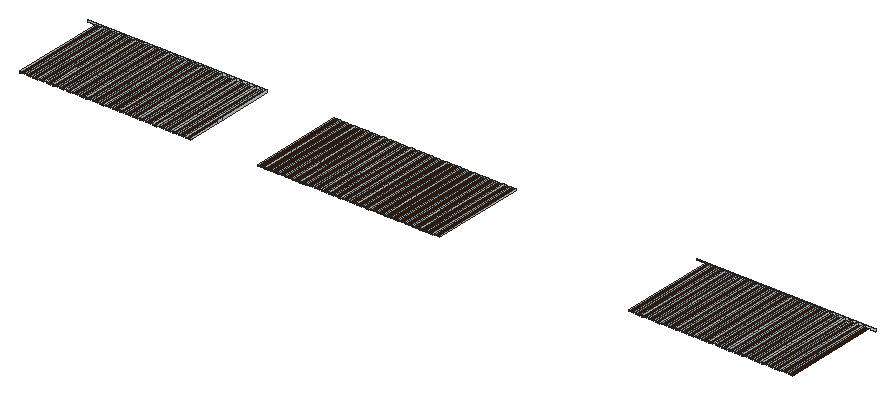
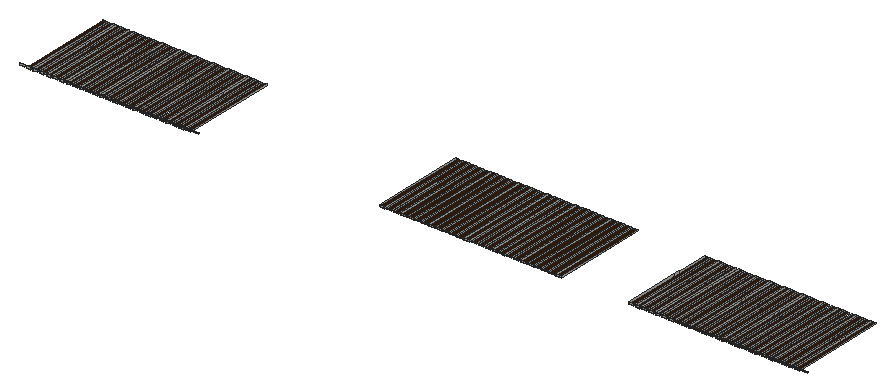
# SketchUp Ruby script. Lengths in inches.
U = 1.inch
M = Sketchup.active_model
def pt(a) = Geom::Point3d.new(a.map { |v| v * U })
def face(e, loops, mat)
  f = e.add_face(loops[0].map { |a| pt(a) })
  loops[1..].each { |l| e.add_face(l.map { |a| pt(a) }).erase! }
  f.material = f.back_material = mat if mat
  f
end
# faces: each face lists its corners as indices into pts; further lists are holes
def faces(e, pts, list, mat = nil) = list.each { |f| face(e, (f[0].is_a?(Array) ? f : [f]).map { |l| l.map { |i| pts[i] } }, mat) }
# xy, xz, yz: faces in a plane at the given z, y or x. An outline is a flat list of corners, or four numbers for a rectangle; further outlines are holes
def ring(l) = l.size == 4 ? [[l[0], l[1]], [l[2], l[1]], [l[2], l[3]], [l[0], l[3]]] : l.each_slice(2).to_a
def flat(e, list, mat, &to3) = list.each { |f| face(e, (f[0].is_a?(Array) ? f : [f]).map { |l| ring(l).map { |u, v| to3.(u, v) } }, mat) }
def xy(e, z, list, mat = nil) = flat(e, list, mat) { |x, y| [x, y, z] }
def xz(e, y, list, mat = nil) = flat(e, list, mat) { |x, z| [x, y, z] }
def yz(e, x, list, mat = nil) = flat(e, list, mat) { |y, z| [x, y, z] }
def lines(e, pts, list) = list.each { |a, b| e.add_line(pt(pts[a]), pt(pts[b])) }
# prism: a flat outline (further loops are holes) pulled along v
def prism(e, loops, v, mat = nil)
  f = face(e, loops, mat); d = Geom::Vector3d.new(v.map { |x| x * U })
  f.pushpull(f.normal.samedirection?(d) ? d.length : -d.length)
end
def box(e, o, s, mat = nil) = prism(e, [[o, [o[0] + s[0], o[1], o[2]], [o[0] + s[0], o[1] + s[1], o[2]], [o[0], o[1] + s[1], o[2]]]], [0, 0, s[2]], mat)
def at(x, y, z, deg = 0) = Geom::Transformation.translation(pt([x, y, z])) * Geom::Transformation.rotation(ORIGIN, Z_AXIS, deg.degrees)
def axes(o, x, y, z) = Geom::Transformation.new([*x, 0, *y, 0, *z, 0, *pt(o).to_a, 1])
def part(name) = M.definitions.add(name)
# library, detail: a bought-in or finely detailed component or shape, given as its bounding box
def library(name, o, s) = part(name).tap { |d| box(d.entities, o, s) }
def detail(e, o, s) = box(e.add_group.entities, o, s)
def put(e, d, t, mat = nil) = e.add_instance(d, t).tap { |i| i.material = mat if mat }
def group(e, t, mat = nil) = e.add_group.tap { |g| g.transformation = t; g.material = mat if mat }.entities
root = M.entities
M.materials.add("[Wood Veneer 01]").color = [51, 28, 15]
xy(root,503.875,[[253.94,246.64,259.43,361.27],[261.94,246.64,267.43,361.27],[269.94,246.64,275.43,361.27],[277.94,246.64,283.43,361.27],[285.94,246.64,291.43,361.27],
  [293.94,246.64,299.43,361.27],[301.94,246.64,307.43,361.27],[309.94,246.64,315.43,361.27],[987.51,246.64,993,361.27],[995.51,246.64,1001,361.27],
  [1003.51,246.64,1009,361.27],[1011.51,246.64,1017,361.27],[1019.51,246.64,1025,361.27],[1027.51,246.64,1033,361.27],[1035.51,246.64,1041,361.27]],"[Wood Veneer 01]")
xy(root,504,[[171.43,283.7,171.43,288.72,172.08,288.63,172.69,288.38,173.21,287.98,173.61,287.46,173.86,286.86,173.94,286.21,173.86,285.56,173.61,284.95,173.21,284.43,172.69,284.03,172.08,283.78],[905,283.7,905,288.72,905.65,288.63,906.25,288.38,906.77,287.98,907.17,287.46,907.42,286.86,907.51,286.21,907.42,285.56,907.17,284.95,906.77,284.43,906.25,284.03,905.65,283.78]])
xy(root,504,[[109.94,246.64,115.43,361.27],[117.94,246.64,123.43,361.27],[125.94,246.64,131.43,361.27],[133.94,246.64,139.43,361.27],[141.94,246.64,147.43,361.27],
  [149.94,246.64,155.43,361.27],[157.94,246.64,163.43,361.27],[165.94,246.64,165.94,361.27,171.43,361.27,171.43,288.72,170.79,288.63,170.18,288.38,169.66,287.98,169.26,287.46,169.01,286.86,168.92,286.21,169.01,285.56,169.26,284.95,169.66,284.43,170.18,284.03,170.79,283.78,171.43,283.7,171.43,246.64],[173.94,246.64,179.43,361.27],[181.94,246.64,187.43,361.27],
  [189.94,246.64,195.43,361.27],[197.94,246.64,203.43,361.27],[205.94,246.64,211.43,361.27],[213.94,246.64,219.43,361.27],[221.94,246.64,227.43,361.27],
  [229.94,246.64,235.43,361.27],[237.94,246.64,243.43,361.27],[245.94,246.64,251.43,361.27],[396.57,246.64,403.28,361.27],[405.07,246.64,411.78,361.27],
  [413.57,246.64,420.28,361.27],[422.07,246.64,428.78,361.27],[430.57,246.64,437.28,361.27],[439.07,246.64,445.78,361.27],[447.57,246.64,454.28,361.27],
  [456.07,246.64,462.78,361.27],[464.57,246.64,471.28,361.27],[473.07,246.64,479.78,361.27],[481.57,246.64,488.28,361.27],[490.07,246.64,496.78,361.27],
  [498.57,246.64,505.28,361.27],[507.07,246.64,513.78,361.27],[515.57,246.64,522.28,361.27],[524.07,246.64,530.78,361.27],[532.57,246.64,539.28,361.27],
  [541.07,246.64,547.78,361.27],[549.57,246.64,556.28,361.27],[558.07,246.64,564.78,361.27],[566.57,246.64,573.28,361.27],[575.07,246.64,581.78,361.27],
  [583.57,246.64,590.28,361.27],[592.07,246.64,598.78,361.27],[600.57,246.64,607.28,361.27],[609.07,246.64,615.78,361.27],[843.51,246.64,849,361.27],
  [851.51,246.64,857,361.27],[859.51,246.64,865,361.27],[867.51,246.64,873,361.27],[875.51,246.64,881,361.27],[883.51,246.64,889,361.27],
  [891.51,246.64,897,361.27],[899.51,246.64,899.51,361.27,905,361.27,905,288.72,904.35,288.63,903.74,288.38,903.22,287.98,902.82,287.46,902.57,286.86,902.49,286.21,902.57,285.56,902.82,284.95,903.22,284.43,903.74,284.03,904.35,283.78,905,283.7,905,246.64],[907.51,246.64,913,361.27],[915.51,246.64,921,361.27],[923.51,246.64,929,361.27],
  [931.51,246.64,937,361.27],[939.51,246.64,945,361.27],[947.51,246.64,953,361.27],[955.51,246.64,961,361.27],[963.51,246.64,969,361.27],
  [971.51,246.64,977,361.27],[979.51,246.64,985,361.27],[171.43,283.7,170.79,283.78,170.18,284.03,169.66,284.43,169.26,284.95,169.01,285.56,168.92,286.21,169.01,286.86,169.26,287.46,169.66,287.98,170.18,288.38,170.79,288.63,171.43,288.72],[905,283.7,904.35,283.78,903.74,284.03,903.22,284.43,902.82,284.95,902.57,285.56,902.49,286.21,902.57,286.86,902.82,287.46,903.22,287.98,903.74,288.38,904.35,288.63,905,288.72]],"[Wood Veneer 01]")
xz(root,246.64,[[253.94,503.875,259.43,505.1875],[261.94,503.875,267.43,503.875,267.43,505.21,261.94,505.19],[269.94,503.875,275.43,503.875,275.43,505.22,269.94,505.21],[277.94,503.875,283.43,503.875,283.43,505.24,277.94,505.23],[285.94,503.875,291.43,503.875,291.43,505.26,285.94,505.25],
  [293.94,503.875,299.43,503.875,299.43,505.28,293.94,505.26],[301.94,503.875,307.43,503.875,307.43,505.29,301.94,505.28],[309.94,503.875,315.43,503.875,315.43,505.3125,309.94,505.3],[987.51,503.875,993,505.1875],[995.51,503.875,1001,503.875,1001,505.21,995.51,505.19],
  [1003.51,503.875,1009,503.875,1009,505.22,1003.51,505.21],[1011.51,503.875,1017,503.875,1017,505.24,1011.51,505.23],[1019.51,503.875,1025,503.875,1025,505.26,1019.51,505.25],[1027.51,503.875,1033,503.875,1033,505.28,1027.51,505.26],[1035.51,503.875,1041,503.875,1041,505.29,1035.51,505.28],
  [109.94,504,115.43,505.3125],[117.94,504,123.43,505.3125],[125.94,504,131.43,505.3125],[133.94,504,139.43,505.3125],[141.94,504,147.43,505.3125],
  [149.94,504,155.43,505.3125],[157.94,504,163.43,505.3125],[165.94,504,171.43,505.3125],[173.94,504,179.43,505.3125],[181.94,504,187.43,505.3125],
  [189.94,504,195.43,505.3125],[197.94,504,203.43,505.3125],[205.94,504,211.43,505.3125],[213.94,504,219.43,505.3125],[221.94,504,227.43,505.3125],
  [229.94,504,235.43,505.3125],[237.94,504,243.43,505.3125],[245.94,504,251.43,505.3125],[396.57,504,403.28,505.3125],[405.07,504,411.78,505.3125],
  [413.57,504,420.28,505.3125],[422.07,504,428.78,505.3125],[430.57,504,437.28,505.3125],[439.07,504,445.78,505.3125],[447.57,504,454.28,505.3125],
  [456.07,504,462.78,505.3125],[464.57,504,471.28,505.3125],[473.07,504,479.78,505.3125],[481.57,504,488.28,505.3125],[490.07,504,496.78,505.3125],
  [498.57,504,505.28,505.3125],[507.07,504,513.78,505.3125],[515.57,504,522.28,505.3125],[524.07,504,530.78,505.3125],[532.57,504,539.28,505.3125],
  [541.07,504,547.78,505.3125],[549.57,504,556.28,505.3125],[558.07,504,564.78,505.3125],[566.57,504,573.28,505.3125],[575.07,504,581.78,505.3125],
  [583.57,504,590.28,505.3125],[592.07,504,598.78,505.3125],[600.57,504,607.28,505.3125],[609.07,504,615.78,505.3125],[843.51,504,849,505.3125],
  [851.51,504,857,505.3125],[859.51,504,865,505.3125],[867.51,504,873,505.3125],[875.51,504,881,505.3125],[883.51,504,889,505.3125],
  [891.51,504,897,505.3125],[899.51,504,905,505.3125],[907.51,504,913,505.3125],[915.51,504,921,505.3125],[923.51,504,929,505.3125],
  [931.51,504,937,505.3125],[939.51,504,945,505.3125],[947.51,504,953,505.3125],[955.51,504,961,505.3125],[963.51,504,969,505.3125],
  [971.51,504,977,505.3125],[979.51,504,985,505.3125]],"[Wood Veneer 01]")
xz(root,361.27,[[261.94,503.875,267.43,503.875,267.43,505.3125,269.94,505.3125,269.94,503.875,275.43,503.875,275.43,505.3125,277.94,505.3125,277.94,503.875,283.43,503.875,283.43,505.3125,285.94,505.3125,285.94,503.875,291.43,503.875,291.43,505.3125,293.94,505.3125,293.94,503.875,299.43,503.875,299.43,505.3125,301.94,505.3125,301.94,503.875,307.43,503.875,307.43,505.3125,309.94,505.3125,309.94,503.875,315.43,503.875,315.43,506.8125,100.18,506.8125,100.18,505.3125,253.94,505.3125,253.94,505.1875,259.43,505.1875,259.43,505.3125,261.94,505.3125],[253.94,503.875,259.43,505.1875],[995.51,503.875,1001,503.875,1001,505.3125,1003.51,505.3125,1003.51,503.875,1009,503.875,1009,505.3125,1011.51,505.3125,1011.51,503.875,1017,503.875,1017,505.3125,1019.51,505.3125,1019.51,503.875,1025,503.875,1025,505.3125,1027.51,505.3125,1027.51,503.875,1033,503.875,1033,505.3125,1035.51,505.3125,1035.51,503.875,1041,503.875,1041,505.3125,1043.51,505.3125,1043.51,503.875,1049,503.875,1049,506.8125,833.74,506.8125,833.74,505.3125,987.51,505.3125,987.51,505.1875,993,505.1875,993,505.3125,995.51,505.3125],[987.51,503.875,993,505.1875],[109.94,504,115.43,505.3125],
  [117.94,504,123.43,505.3125],[125.94,504,131.43,505.3125],[133.94,504,139.43,505.3125],[141.94,504,147.43,505.3125],[149.94,504,155.43,505.3125],
  [157.94,504,163.43,505.3125],[165.94,504,171.43,505.3125],[173.94,504,179.43,505.3125],[181.94,504,187.43,505.3125],[189.94,504,195.43,505.3125],
  [197.94,504,203.43,505.3125],[205.94,504,211.43,505.3125],[213.94,504,219.43,505.3125],[221.94,504,227.43,505.3125],[229.94,504,235.43,505.3125],
  [237.94,504,243.43,505.3125],[245.94,504,251.43,505.3125],[396.57,504,403.28,505.3125],[405.07,504,411.78,505.3125],[413.57,504,420.28,505.3125],
  [422.07,504,428.78,505.3125],[430.57,504,437.28,505.3125],[439.07,504,445.78,505.3125],[447.57,504,454.28,505.3125],[456.07,504,462.78,505.3125],
  [464.57,504,471.28,505.3125],[473.07,504,479.78,505.3125],[481.57,504,488.28,505.3125],[490.07,504,496.78,505.3125],[498.57,504,505.28,505.3125],
  [507.07,504,513.78,505.3125],[515.57,504,522.28,505.3125],[524.07,504,530.78,505.3125],[532.57,504,539.28,505.3125],[541.07,504,547.78,505.3125],
  [549.57,504,556.28,505.3125],[558.07,504,564.78,505.3125],[566.57,504,573.28,505.3125],[575.07,504,581.78,505.3125],[583.57,504,590.28,505.3125],
  [592.07,504,598.78,505.3125],[600.57,504,607.28,505.3125],[609.07,504,614.76,505.3125],[614.76,504,615.78,505.3125],[843.51,504,849,505.3125],
  [851.51,504,857,505.3125],[859.51,504,865,505.3125],[867.51,504,873,505.3125],[875.51,504,881,505.3125],[883.51,504,889,505.3125],
  [891.51,504,897,505.3125],[899.51,504,905,505.3125],[907.51,504,913,505.3125],[915.51,504,921,505.3125],[923.51,504,929,505.3125],
  [931.51,504,937,505.3125],[939.51,504,945,505.3125],[947.51,504,953,505.3125],[955.51,504,961,505.3125],[963.51,504,969,505.3125],
  [971.51,504,977,505.3125],[979.51,504,985,505.3125]])
yz(root,109.94,[[246.64,504,361.27,505.3125]])
yz(root,115.43,[[246.64,504,286.21,505.3125],[286.21,504,293.45,505.3125],[293.45,504,293.46,505.3125],[293.46,504,361.27,505.3125]])
yz(root,117.94,[[246.64,504,361.27,505.3125]])
yz(root,123.43,[[246.64,504,286.21,505.3125],[286.21,504,293.45,505.3125],[293.45,504,293.46,505.3125],[293.46,504,361.27,505.3125]])
yz(root,125.94,[[246.64,504,361.27,505.3125]])
yz(root,131.43,[[246.64,504,286.21,505.3125],[286.21,504,293.45,505.3125],[293.45,504,293.46,505.3125],[293.46,504,361.27,505.3125]])
yz(root,133.94,[[246.64,504,361.27,505.3125]])
yz(root,139.43,[[246.64,504,286.21,505.3125],[286.21,504,293.45,505.3125],[293.45,504,293.46,505.3125],[293.46,504,361.27,505.3125]])
yz(root,141.94,[[246.64,504,361.27,505.3125]])
yz(root,147.43,[[246.64,504,286.21,505.3125],[286.21,504,293.45,505.3125],[293.45,504,293.46,505.3125],[293.46,504,361.27,505.3125]])
yz(root,149.94,[[246.64,504,361.27,505.3125]])
yz(root,155.43,[[246.64,504,286.21,505.3125],[286.21,504,293.45,505.3125],[293.45,504,293.46,505.3125],[293.46,504,361.27,505.3125]])
yz(root,157.94,[[246.64,504,361.27,505.3125]])
yz(root,163.43,[[246.64,504,286.21,505.3125],[286.21,504,293.45,505.3125],[293.45,504,293.46,505.3125],[293.46,504,361.27,505.3125]])
yz(root,165.94,[[246.64,504,361.27,505.3125]])
yz(root,171.43,[[246.64,504,286.21,505.3125],[286.21,504,293.45,505.3125],[293.45,504,293.46,505.3125],[293.46,504,361.27,505.3125]])
yz(root,173.94,[[246.64,504,361.27,505.3125]])
yz(root,179.43,[[246.64,504,286.21,505.3125],[286.21,504,293.45,505.3125],[293.45,504,293.46,505.3125],[293.46,504,361.27,505.3125]])
yz(root,181.94,[[246.64,504,361.27,505.3125]])
yz(root,187.43,[[246.64,504,286.21,505.3125],[286.21,504,293.45,505.3125],[293.45,504,293.46,505.3125],[293.46,504,361.27,505.3125]])
yz(root,189.94,[[246.64,504,361.27,505.3125]])
yz(root,195.43,[[246.64,504,286.21,505.3125],[286.21,504,293.45,505.3125],[293.45,504,293.46,505.3125],[293.46,504,361.27,505.3125]])
yz(root,197.94,[[246.64,504,361.27,505.3125]])
yz(root,203.43,[[246.64,504,286.21,505.3125],[286.21,504,293.45,505.3125],[293.45,504,293.46,505.3125],[293.46,504,361.27,505.3125]])
yz(root,205.94,[[246.64,504,361.27,505.3125]])
yz(root,211.43,[[246.64,504,286.21,505.3125],[286.21,504,293.45,505.3125],[293.45,504,293.46,505.3125],[293.46,504,361.27,505.3125]])
yz(root,213.94,[[246.64,504,361.27,505.3125]])
yz(root,219.43,[[246.64,504,286.21,505.3125],[286.21,504,293.45,505.3125],[293.45,504,293.46,505.3125],[293.46,504,361.27,505.3125]])
yz(root,221.94,[[246.64,504,361.27,505.3125]])
yz(root,227.43,[[246.64,504,286.21,505.3125],[286.21,504,293.45,505.3125],[293.45,504,293.46,505.3125],[293.46,504,361.27,505.3125]])
yz(root,229.94,[[246.64,504,361.27,505.3125]])
yz(root,235.43,[[246.64,504,286.21,505.3125],[286.21,504,293.45,505.3125],[293.45,504,293.46,505.3125],[293.46,504,361.27,505.3125]])
yz(root,237.94,[[246.64,504,361.27,505.3125]])
yz(root,243.43,[[246.64,504,286.21,505.3125],[286.21,504,293.45,505.3125],[293.45,504,293.46,505.3125],[293.46,504,361.27,505.3125]])
yz(root,245.94,[[246.64,504,361.27,505.3125]])
yz(root,251.43,[[246.64,504,286.21,505.3125],[286.21,504,293.45,505.3125],[293.45,504,293.46,505.3125],[293.46,504,361.27,505.3125]])
yz(root,253.94,[[246.64,503.875,361.27,505.1875]])
yz(root,259.43,[[246.64,503.875,286.21,505.1875],[286.21,503.875,293.45,505.1875],[293.45,503.875,293.46,505.1875],[293.46,503.875,361.27,505.1875]])
yz(root,261.94,[[246.64,503.875,361.27,505.3125]])
yz(root,267.43,[[246.64,503.875,286.21,505.3125],[286.21,503.875,293.45,505.3125],[293.45,503.875,293.46,505.3125],[293.46,503.875,361.27,505.3125]])
yz(root,269.94,[[246.64,503.875,361.27,505.3125]])
yz(root,275.43,[[246.64,503.875,286.21,505.3125],[286.21,503.875,293.45,505.3125],[293.45,503.875,293.46,505.3125],[293.46,503.875,361.27,505.3125]])
yz(root,277.94,[[246.64,503.875,361.27,505.3125]])
yz(root,283.43,[[246.64,503.875,286.21,505.3125],[286.21,503.875,293.45,505.3125],[293.45,503.875,293.46,505.3125],[293.46,503.875,361.27,505.3125]])
yz(root,285.94,[[246.64,503.875,361.27,505.3125]])
yz(root,291.43,[[246.64,503.875,286.21,505.3125],[286.21,503.875,293.45,505.3125],[293.45,503.875,293.46,505.3125],[293.46,503.875,361.27,505.3125]])
yz(root,293.94,[[246.64,503.875,361.27,505.3125]])
yz(root,299.43,[[246.64,503.875,286.21,505.3125],[286.21,503.875,293.45,505.3125],[293.45,503.875,293.46,505.3125],[293.46,503.875,361.27,505.3125]])
yz(root,301.94,[[246.64,503.875,361.27,505.3125]])
yz(root,307.43,[[246.64,503.875,286.21,505.3125],[286.21,503.875,293.45,505.3125],[293.45,503.875,293.46,505.3125],[293.46,503.875,361.27,505.3125]])
yz(root,309.94,[[246.64,503.875,361.27,505.3125]])
yz(root,315.43,[[246.64,503.875,286.21,505.3125],[286.21,503.875,293.45,506.8125],[293.45,503.875,293.46,506.8125],[293.46,503.875,361.27,506.8125]])
yz(root,396.57,[[246.64,504,286.21,505.3125],[286.21,504,293.45,505.3125],[293.45,504,361.27,505.3125]])
yz(root,403.28,[[246.64,504,361.27,505.3125]])
yz(root,405.07,[[246.64,504,286.21,505.3125],[286.21,504,293.45,505.3125],[293.45,504,361.27,505.3125]])
yz(root,411.78,[[246.64,504,361.27,505.3125]])
yz(root,413.57,[[246.64,504,286.21,505.3125],[286.21,504,293.45,505.3125],[293.45,504,361.27,505.3125]])
yz(root,420.28,[[246.64,504,361.27,505.3125]])
yz(root,422.07,[[246.64,504,286.21,505.3125],[286.21,504,293.45,505.3125],[293.45,504,361.27,505.3125]])
yz(root,428.78,[[246.64,504,361.27,505.3125]])
yz(root,430.57,[[246.64,504,286.21,505.3125],[286.21,504,293.45,505.3125],[293.45,504,361.27,505.3125]])
yz(root,437.28,[[246.64,504,361.27,505.3125]])
yz(root,439.07,[[246.64,504,286.21,505.3125],[286.21,504,293.45,505.3125],[293.45,504,361.27,505.3125]])
yz(root,445.78,[[246.64,504,361.27,505.3125]])
yz(root,447.57,[[246.64,504,286.21,505.3125],[286.21,504,293.45,505.3125],[293.45,504,361.27,505.3125]])
yz(root,454.28,[[246.64,504,361.27,505.3125]])
yz(root,456.07,[[246.64,504,286.21,505.3125],[286.21,504,293.45,505.3125],[293.45,504,361.27,505.3125]])
yz(root,462.78,[[246.64,504,361.27,505.3125]])
yz(root,464.57,[[246.64,504,286.21,505.3125],[286.21,504,293.45,505.3125],[293.45,504,361.27,505.3125]])
yz(root,471.28,[[246.64,504,361.27,505.3125]])
yz(root,473.07,[[246.64,504,286.21,505.3125],[286.21,504,293.45,505.3125],[293.45,504,361.27,505.3125]])
yz(root,479.78,[[246.64,504,361.27,505.3125]])
yz(root,481.57,[[246.64,504,286.21,505.3125],[286.21,504,293.45,505.3125],[293.45,504,361.27,505.3125]])
yz(root,488.28,[[246.64,504,361.27,505.3125]])
yz(root,490.07,[[246.64,504,286.21,505.3125],[286.21,504,293.45,505.3125],[293.45,504,361.27,505.3125]])
yz(root,496.78,[[246.64,504,361.27,505.3125]])
yz(root,498.57,[[246.64,504,286.21,505.3125],[286.21,504,293.45,505.3125],[293.45,504,361.27,505.3125]])
yz(root,505.28,[[246.64,504,361.27,505.3125]])
yz(root,507.07,[[246.64,504,286.21,505.3125],[286.21,504,293.45,505.3125],[293.45,504,361.27,505.3125]])
yz(root,513.78,[[246.64,504,361.27,505.3125]])
yz(root,515.57,[[246.64,504,286.21,505.3125],[286.21,504,293.45,505.3125],[293.45,504,361.27,505.3125]])
yz(root,522.28,[[246.64,504,361.27,505.3125]])
yz(root,524.07,[[246.64,504,286.21,505.3125],[286.21,504,293.45,505.3125],[293.45,504,361.27,505.3125]])
yz(root,530.78,[[246.64,504,361.27,505.3125]])
yz(root,532.57,[[246.64,504,286.21,505.3125],[286.21,504,293.45,505.3125],[293.45,504,361.27,505.3125]])
yz(root,539.28,[[246.64,504,361.27,505.3125]])
yz(root,541.07,[[246.64,504,286.21,505.3125],[286.21,504,293.45,505.3125],[293.45,504,361.27,505.3125]])
yz(root,547.78,[[246.64,504,361.27,505.3125]])
yz(root,549.57,[[246.64,504,286.21,505.3125],[286.21,504,293.45,505.3125],[293.45,504,361.27,505.3125]])
yz(root,556.28,[[246.64,504,361.27,505.3125]])
yz(root,558.07,[[246.64,504,286.21,505.3125],[286.21,504,293.45,505.3125],[293.45,504,361.27,505.3125]])
yz(root,564.78,[[246.64,504,361.27,505.3125]])
yz(root,566.57,[[246.64,504,286.21,505.3125],[286.21,504,293.45,505.3125],[293.45,504,361.27,505.3125]])
yz(root,573.28,[[246.64,504,361.27,505.3125]])
yz(root,575.07,[[246.64,504,286.21,505.3125],[286.21,504,293.45,505.3125],[293.45,504,361.27,505.3125]])
yz(root,581.78,[[246.64,504,361.27,505.3125]])
yz(root,583.57,[[246.64,504,286.21,505.3125],[286.21,504,293.45,505.3125],[293.45,504,361.27,505.3125]])
yz(root,590.28,[[246.64,504,361.27,505.3125]])
yz(root,592.07,[[246.64,504,286.21,505.3125],[286.21,504,293.45,505.3125],[293.45,504,361.27,505.3125]])
yz(root,598.78,[[246.64,504,361.27,505.3125]])
yz(root,600.57,[[246.64,504,286.21,505.3125],[286.21,504,293.45,505.3125],[293.45,504,361.27,505.3125]])
yz(root,607.28,[[246.64,504,361.27,505.3125]])
yz(root,609.07,[[246.64,504,286.21,505.3125],[286.21,504,293.45,505.3125],[293.45,504,361.27,505.3125]])
yz(root,615.78,[[246.64,504,361.27,505.3125]])
yz(root,843.51,[[246.64,504,361.27,505.3125]])
yz(root,849,[[246.64,504,286.21,505.3125],[286.21,504,293.45,505.3125],[293.45,504,293.46,505.3125],[293.46,504,361.27,505.3125]])
yz(root,851.51,[[246.64,504,361.27,505.3125]])
yz(root,857,[[246.64,504,286.21,505.3125],[286.21,504,293.45,505.3125],[293.45,504,293.46,505.3125],[293.46,504,361.27,505.3125]])
yz(root,859.51,[[246.64,504,361.27,505.3125]])
yz(root,865,[[246.64,504,286.21,505.3125],[286.21,504,293.45,505.3125],[293.45,504,293.46,505.3125],[293.46,504,361.27,505.3125]])
yz(root,867.51,[[246.64,504,361.27,505.3125]])
yz(root,873,[[246.64,504,286.21,505.3125],[286.21,504,293.45,505.3125],[293.45,504,293.46,505.3125],[293.46,504,361.27,505.3125]])
yz(root,875.51,[[246.64,504,361.27,505.3125]])
yz(root,881,[[246.64,504,286.21,505.3125],[286.21,504,293.45,505.3125],[293.45,504,293.46,505.3125],[293.46,504,361.27,505.3125]])
yz(root,883.51,[[246.64,504,361.27,505.3125]])
yz(root,889,[[246.64,504,286.21,505.3125],[286.21,504,293.45,505.3125],[293.45,504,293.46,505.3125],[293.46,504,361.27,505.3125]])
yz(root,891.51,[[246.64,504,361.27,505.3125]])
yz(root,897,[[246.64,504,286.21,505.3125],[286.21,504,293.45,505.3125],[293.45,504,293.46,505.3125],[293.46,504,361.27,505.3125]])
yz(root,899.51,[[246.64,504,361.27,505.3125]])
yz(root,905,[[246.64,504,286.21,505.3125],[286.21,504,293.45,505.3125],[293.45,504,293.46,505.3125],[293.46,504,361.27,505.3125]])
yz(root,907.51,[[246.64,504,361.27,505.3125]])
yz(root,913,[[246.64,504,286.21,505.3125],[286.21,504,293.45,505.3125],[293.45,504,293.46,505.3125],[293.46,504,361.27,505.3125]])
yz(root,915.51,[[246.64,504,361.27,505.3125]])
yz(root,921,[[246.64,504,286.21,505.3125],[286.21,504,293.45,505.3125],[293.45,504,293.46,505.3125],[293.46,504,361.27,505.3125]])
yz(root,923.51,[[246.64,504,361.27,505.3125]])
yz(root,929,[[246.64,504,286.21,505.3125],[286.21,504,293.45,505.3125],[293.45,504,293.46,505.3125],[293.46,504,361.27,505.3125]])
yz(root,931.51,[[246.64,504,361.27,505.3125]])
yz(root,937,[[246.64,504,286.21,505.3125],[286.21,504,293.45,505.3125],[293.45,504,293.46,505.3125],[293.46,504,361.27,505.3125]])
yz(root,939.51,[[246.64,504,361.27,505.3125]])
yz(root,945,[[246.64,504,286.21,505.3125],[286.21,504,293.45,505.3125],[293.45,504,293.46,505.3125],[293.46,504,361.27,505.3125]])
yz(root,947.51,[[246.64,504,361.27,505.3125]])
yz(root,953,[[246.64,504,286.21,505.3125],[286.21,504,293.45,505.3125],[293.45,504,293.46,505.3125],[293.46,504,361.27,505.3125]])
yz(root,955.51,[[246.64,504,361.27,505.3125]])
yz(root,961,[[246.64,504,286.21,505.3125],[286.21,504,293.45,505.3125],[293.45,504,293.46,505.3125],[293.46,504,361.27,505.3125]])
yz(root,963.51,[[246.64,504,361.27,505.3125]])
yz(root,969,[[246.64,504,286.21,505.3125],[286.21,504,293.45,505.3125],[293.45,504,293.46,505.3125],[293.46,504,361.27,505.3125]])
yz(root,971.51,[[246.64,504,361.27,505.3125]])
yz(root,977,[[246.64,504,286.21,505.3125],[286.21,504,293.45,505.3125],[293.45,504,293.46,505.3125],[293.46,504,361.27,505.3125]])
yz(root,979.51,[[246.64,504,361.27,505.3125]])
yz(root,985,[[246.64,504,286.21,505.3125],[286.21,504,293.45,505.3125],[293.45,504,293.46,505.3125],[293.46,504,361.27,505.3125]])
yz(root,987.51,[[246.64,503.875,361.27,505.1875]])
yz(root,993,[[246.64,503.875,286.21,505.1875],[286.21,503.875,293.45,505.1875],[293.45,503.875,293.46,505.1875],[293.46,503.875,361.27,505.1875]])
yz(root,995.51,[[246.64,503.875,361.27,505.3125]])
yz(root,1001,[[246.64,503.875,286.21,505.3125],[286.21,503.875,293.45,505.3125],[293.45,503.875,293.46,505.3125],[293.46,503.875,361.27,505.3125]])
yz(root,1003.51,[[246.64,503.875,361.27,505.3125]])
yz(root,1009,[[246.64,503.875,286.21,505.3125],[286.21,503.875,293.45,505.3125],[293.45,503.875,293.46,505.3125],[293.46,503.875,361.27,505.3125]])
yz(root,1011.51,[[246.64,503.875,361.27,505.3125]])
yz(root,1017,[[246.64,503.875,286.21,505.3125],[286.21,503.875,293.45,505.3125],[293.45,503.875,293.46,505.3125],[293.46,503.875,361.27,505.3125]])
yz(root,1019.51,[[246.64,503.875,361.27,505.3125]])
yz(root,1025,[[246.64,503.875,286.21,505.3125],[286.21,503.875,293.45,505.3125],[293.45,503.875,293.46,505.3125],[293.46,503.875,361.27,505.3125]])
yz(root,1027.51,[[246.64,503.875,361.27,505.3125]])
yz(root,1033,[[246.64,503.875,286.21,505.3125],[286.21,503.875,293.45,505.3125],[293.45,503.875,293.46,505.3125],[293.46,503.875,361.27,505.3125]])
yz(root,1035.51,[[246.64,503.875,361.27,505.3125]])
